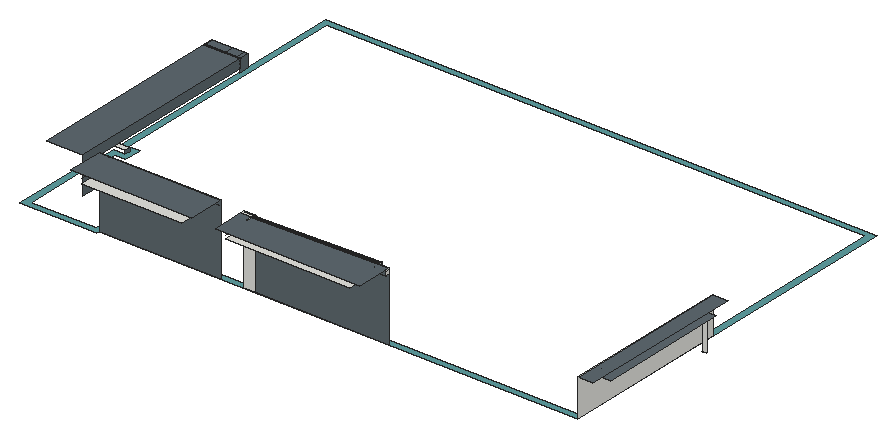
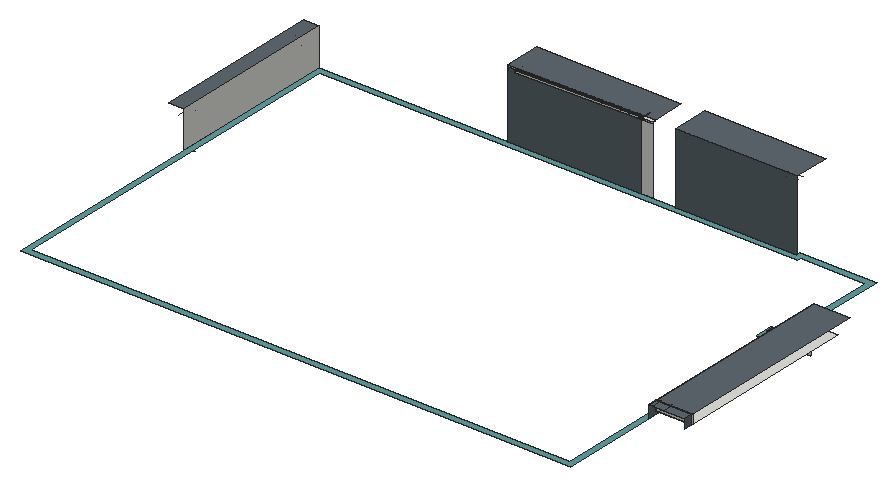
# SketchUp Ruby script. Lengths in inches.
U = 1.inch
M = Sketchup.active_model
def pt(a) = Geom::Point3d.new(a.map { |v| v * U })
def face(e, loops, mat)
  f = e.add_face(loops[0].map { |a| pt(a) })
  loops[1..].each { |l| e.add_face(l.map { |a| pt(a) }).erase! }
  f.material = f.back_material = mat if mat
  f
end
# faces: each face lists its corners as indices into pts; further lists are holes
def faces(e, pts, list, mat = nil) = list.each { |f| face(e, (f[0].is_a?(Array) ? f : [f]).map { |l| l.map { |i| pts[i] } }, mat) }
# xy, xz, yz: faces in a plane at the given z, y or x. An outline is a flat list of corners, or four numbers for a rectangle; further outlines are holes
def ring(l) = l.size == 4 ? [[l[0], l[1]], [l[2], l[1]], [l[2], l[3]], [l[0], l[3]]] : l.each_slice(2).to_a
def flat(e, list, mat, &to3) = list.each { |f| face(e, (f[0].is_a?(Array) ? f : [f]).map { |l| ring(l).map { |u, v| to3.(u, v) } }, mat) }
def xy(e, z, list, mat = nil) = flat(e, list, mat) { |x, y| [x, y, z] }
def xz(e, y, list, mat = nil) = flat(e, list, mat) { |x, z| [x, y, z] }
def yz(e, x, list, mat = nil) = flat(e, list, mat) { |y, z| [x, y, z] }
def lines(e, pts, list) = list.each { |a, b| e.add_line(pt(pts[a]), pt(pts[b])) }
# prism: a flat outline (further loops are holes) pulled along v
def prism(e, loops, v, mat = nil)
  f = face(e, loops, mat); d = Geom::Vector3d.new(v.map { |x| x * U })
  f.pushpull(f.normal.samedirection?(d) ? d.length : -d.length)
end
def box(e, o, s, mat = nil) = prism(e, [[o, [o[0] + s[0], o[1], o[2]], [o[0] + s[0], o[1] + s[1], o[2]], [o[0], o[1] + s[1], o[2]]]], [0, 0, s[2]], mat)
def at(x, y, z, deg = 0) = Geom::Transformation.translation(pt([x, y, z])) * Geom::Transformation.rotation(ORIGIN, Z_AXIS, deg.degrees)
def axes(o, x, y, z) = Geom::Transformation.new([*x, 0, *y, 0, *z, 0, *pt(o).to_a, 1])
def part(name) = M.definitions.add(name)
# library, detail: a bought-in or finely detailed component or shape, given as its bounding box
def library(name, o, s) = part(name).tap { |d| box(d.entities, o, s) }
def detail(e, o, s) = box(e.add_group.entities, o, s)
def put(e, d, t, mat = nil) = e.add_instance(d, t).tap { |i| i.material = mat if mat }
def group(e, t, mat = nil) = e.add_group.tap { |g| g.transformation = t; g.material = mat if mat }.entities
root = M.entities
M.materials.add("[0081_CadetBlue]").color = [95, 158, 160]
M.materials.add("[Formica Speckled Grey]").color = [94, 105, 111]
xy(root,684.183,[[[77.814,152.582,200.97,152.582,200.97,158.582,972.467,158.582,972.467,761.484,83.814,761.484,83.814,342.404,101.939,342.404,101.939,333.733,83.814,333.733,83.814,271.699,77.814,271.699],[86.814,161.582,86.814,262.699,92.814,262.699,92.814,324.733,110.939,324.733,110.939,351.404,92.814,351.404,92.814,752.484,963.467,752.484,963.467,167.582,191.97,167.582,191.97,161.582]]],"[0081_CadetBlue]")
xy(root,689.85,[[26.029,295.241,26.029,589.716,83.814,589.716,83.814,587.654,68.814,587.654,68.814,578.983,74.814,578.983,74.814,573.966,68.814,573.966,68.814,565.295,74.814,565.295,74.814,560.279,68.814,560.279,68.814,551.608,74.814,551.608,74.814,546.591,68.814,546.591,68.814,537.92,74.814,537.92,74.814,532.904,68.814,532.904,68.814,524.233,74.814,524.233,74.814,519.216,68.814,519.216,68.814,510.545,74.814,510.545,74.814,505.529,68.814,505.529,68.814,496.858,74.814,496.858,74.814,491.841,68.814,491.841,68.814,483.17,74.814,483.17,74.814,478.154,68.814,478.154,68.814,469.483,74.814,469.483,74.814,464.466,68.814,464.466,68.814,455.795,74.814,455.795,74.814,450.779,68.814,450.779,68.814,442.108,74.814,442.108,74.814,437.091,68.814,437.091,68.814,428.42,74.814,428.42,74.814,423.404,68.814,423.404,68.814,414.733,74.814,414.733,74.814,409.716,68.814,409.716,68.814,401.045,74.814,401.045,74.814,396.029,68.814,396.029,68.814,387.358,74.814,387.358,74.814,382.341,68.814,382.341,68.814,373.67,74.814,373.67,74.814,369.029,68.814,369.029,68.814,360.358,74.814,360.358,74.814,355.716,68.814,355.716,68.814,347.045,74.814,347.045,74.814,342.404,68.814,342.404,68.814,333.733,74.814,333.733,74.814,329.091,68.814,329.091,68.814,320.42,74.814,320.42,74.814,315.779,68.814,315.779,68.814,307.108,74.814,307.108,74.814,302.466,68.814,302.466,68.814,295.241],[68.814,295.241,74.814,302.466],[74.814,295.241,83.814,333.733],[68.814,307.108,74.814,315.779],[68.814,320.42,74.814,329.091],
  [68.814,333.733,74.814,342.404],[74.814,333.733,83.814,342.404],[83.814,333.733,101.939,342.404],[74.814,342.404,83.814,587.654],[68.814,347.045,74.814,355.716],
  [68.814,360.358,74.814,369.029],[68.814,373.67,74.814,382.341],[68.814,387.358,74.814,396.029],[68.814,401.045,74.814,409.716],[68.814,414.733,74.814,423.404],
  [68.814,428.42,74.814,437.091],[68.814,442.108,74.814,450.779],[68.814,455.795,74.814,464.466],[68.814,469.483,74.814,478.154],[68.814,483.17,74.814,491.841],
  [68.814,496.858,74.814,505.529],[68.814,510.545,74.814,519.216],[68.814,524.233,74.814,532.904],[68.814,537.92,74.814,546.591],[68.814,551.608,74.814,560.279],
  [68.814,565.295,74.814,573.966],[68.814,578.983,74.814,587.654]])
xy(root,704.683,[[26.029,271.699,83.814,587.654],[26.029,587.654,59.814,589.716],[59.814,587.654,77.814,589.716],[77.814,587.654,83.814,589.716],[26.029,589.716,59.814,604.3125],
  [59.814,589.716,77.814,604.3125],[77.814,589.716,83.814,604.3125]],"[Formica Speckled Grey]")
xy(root,732.183,[[974.717,194.926,980.717,205.629],[975.029,210.613,980.717,221.317],[975.029,226.301,980.717,237.004],[975.029,241.988,980.717,252.692],[975.029,257.676,980.717,268.379],
  [975.029,273.363,980.717,284.067],[975.029,289.051,980.717,299.754],[975.029,304.738,980.717,315.442],[975.029,320.426,980.717,331.129],[975.029,336.113,980.717,346.817],
  [975.029,351.801,981.029,362.504],[975.029,367.488,981.029,378.192],[975.029,383.176,981.029,393.879],[975.029,398.863,981.029,408.529]])
xy(root,732.183,[[980.717,194.926,980.717,205.629,975.029,205.629,975.029,210.613,980.717,210.613,980.717,221.317,975.029,221.317,975.029,226.301,980.717,226.301,980.717,237.004,975.029,237.004,975.029,241.988,980.717,241.988,980.717,252.692,975.029,252.692,975.029,257.676,980.717,257.676,980.717,268.379,975.029,268.379,975.029,273.363,980.717,273.363,980.717,284.067,975.029,284.067,975.029,289.051,980.717,289.051,980.717,299.754,975.029,299.754,975.029,304.738,980.717,304.738,980.717,315.442,975.029,315.442,975.029,320.426,980.717,320.426,980.717,331.129,975.029,331.129,975.029,336.113,980.717,336.113,980.717,346.817,975.029,346.817,975.029,351.801,981.029,351.801,981.029,362.504,975.029,362.504,975.029,367.488,981.029,367.488,981.029,378.192,975.029,378.192,975.029,383.176,981.029,383.176,981.029,393.879,975.029,393.879,975.029,398.863,981.029,398.863,981.029,408.529,996.467,408.529,996.467,194.926]],"[Formica Speckled Grey]")
xy(root,744.183,[[972.467,158.582,996.467,431.225]],"[Formica Speckled Grey]")
xy(root,784.183,[[217.792,100.797,217.792,140.582,223.26,140.582,223.26,137.582,231.22,137.582,231.22,140.582,235.635,140.582,235.635,137.582,243.595,137.582,243.595,140.582,248.01,140.582,248.01,137.582,255.97,137.582,255.97,140.582,260.385,140.582,260.385,137.582,268.345,137.582,268.345,140.582,272.76,140.582,272.76,137.582,280.72,137.582,280.72,140.582,285.135,140.582,285.135,137.582,293.095,137.582,293.095,140.582,297.51,140.582,297.51,137.582,305.47,137.582,305.47,140.582,309.885,140.582,309.885,137.582,317.845,137.582,317.845,140.582,322.26,140.582,322.26,137.582,330.22,137.582,330.22,140.582,334.635,140.582,334.635,137.582,342.595,137.582,342.595,140.582,347.01,140.582,347.01,137.582,354.97,137.582,354.97,140.582,359.385,140.582,359.385,137.582,367.345,137.582,367.345,140.582,371.76,140.582,371.76,137.582,379.72,137.582,379.72,100.797],[223.26,137.582,231.22,140.582],[235.635,137.582,243.595,140.582],[248.01,137.582,255.97,140.582],[260.385,137.582,268.345,140.582],
  [272.76,137.582,280.72,140.582],[285.135,137.582,293.095,140.582],[297.51,137.582,305.47,140.582],[309.885,137.582,317.845,140.582],[322.26,137.582,330.22,140.582],
  [334.635,137.582,342.595,140.582],[347.01,137.582,354.97,140.582],[359.385,137.582,367.345,140.582],[371.76,137.582,379.72,140.582],[217.792,140.582,217.792,143.582,379.72,143.582,379.72,140.582,305.47,140.582,305.47,140.894,297.51,140.894,297.51,140.582],
  [297.51,140.582,305.47,140.894],[217.792,143.582,379.72,146.582],[217.792,146.582,379.72,155.582]])
xy(root,786.183,[[450.855,100.797,450.855,152.582,451.124,143.586,451.214,140.587,460.874,140.877,460.784,143.875,651.119,149.574,651.119,143.76,645.312,143.586,645.388,141.034,651.119,141.206,651.119,100.797],[451.214,140.587,451.124,143.586,460.784,143.875,460.874,140.877],[645.388,141.034,645.312,143.586,651.119,143.76,651.119,141.206],[651.119,141.206,651.196,141.208,651.119,143.76],[651.196,141.208,655.048,141.323,654.971,143.875,651.119,143.76],
  [651.119,149.574,651.235,149.578,651.504,149.586,651.417,152.508,651.119,152.508]])
xy(root,792.183,[[451.124,143.586,651.235,149.578,650.967,158.523,450.856,152.531],[651.235,149.578,651.235,158.531,650.967,158.523],[651.235,149.578,651.235,158.531,651.237,158.531,651.504,149.586],[651.504,149.586,651.237,158.531,651.592,158.542,651.86,149.597],[668.057,152.508,668.057,158.519,667.692,152.53],
  [450.856,152.531,650.967,158.523,650.965,158.582,527.197,158.582,450.855,156.296,450.855,152.582],[450.855,152.582,450.744,156.293,450.855,156.296],[450.744,156.293,450.706,157.542,450.817,157.545,450.855,156.296],[450.855,156.296,450.817,157.545,450.855,157.547],[450.855,156.296,527.197,158.582,485.433,158.582,450.855,157.547],
  [450.706,157.542,450.682,158.354,450.793,158.358,450.817,157.545],[450.817,157.545,450.793,158.358,450.83,158.359,450.855,157.547],[450.855,157.547,450.83,158.359,450.855,158.359],[450.855,157.547,485.433,158.582,458.286,158.582,450.855,158.359],[450.855,158.359,458.286,158.582,450.855,158.582],
  [668.057,158.519,668.057,158.582,668.053,158.52],[650.967,158.523,650.965,158.582,651.233,158.582,651.235,158.531],[650.967,158.523,651.235,158.531,651.235,158.582,650.965,158.582],[651.235,158.531,651.233,158.582,651.235,158.582,651.237,158.531],[651.235,158.531,651.237,158.531,651.235,158.582],
  [651.237,158.531,651.235,158.582,651.591,158.582,651.592,158.542],[458.286,158.582,485.409,159.394,485.433,158.582],[485.433,158.582,485.409,159.394,527.136,160.644,527.16,159.831],[485.433,158.582,527.16,159.831,527.197,158.582],[527.197,158.582,527.16,159.831,650.817,163.534,650.855,162.285],
  [527.197,158.582,650.855,162.285,650.965,158.582],[650.965,158.582,650.855,162.285,651.122,162.293,651.233,158.582],[651.233,158.582,651.122,162.293,651.124,162.293,651.235,158.582],[651.235,158.582,651.124,162.293,651.479,162.303,651.591,158.582],[527.16,159.831,527.136,160.644,650.793,164.346,650.817,163.534],
  [650.855,162.285,650.817,163.534,651.085,163.542,651.122,162.293],[651.122,162.293,651.085,163.542,651.086,163.542,651.124,162.293],[651.124,162.293,651.086,163.542,651.442,163.553,651.479,162.303],[650.817,163.534,650.793,164.346,651.061,164.354,651.085,163.542],[651.085,163.542,651.061,164.354,651.062,164.354,651.086,163.542],
  [651.086,163.542,651.062,164.354,651.417,164.365,651.442,163.553]])
xy(root,795.183,[[450.856,152.531,651.237,158.531,651.235,158.582,651.124,162.293,450.855,156.296,450.855,152.582],[434.033,152.582,450.855,152.582,450.744,156.293,450.706,157.542,450.682,158.354,450.793,158.358,450.83,158.359,450.855,158.359,450.855,158.582,434.033,158.582],[450.855,152.582,450.855,156.296,450.744,156.293],[450.744,156.293,450.855,156.296,450.817,157.545,450.706,157.542],[450.855,156.296,450.855,157.547,450.817,157.545],
  [450.855,156.296,651.124,162.293,651.086,163.542,450.855,157.547],[450.706,157.542,450.817,157.545,450.793,158.358,450.682,158.354],[450.817,157.545,450.855,157.547,450.83,158.359,450.793,158.358],[450.855,157.547,450.855,158.359,450.83,158.359],[450.855,157.547,651.086,163.542,651.062,164.354,450.855,158.359],
  [651.237,158.531,651.592,158.542,651.591,158.582,651.235,158.582],[651.235,158.582,651.591,158.582,651.479,162.303,651.124,162.293],[651.124,162.293,651.479,162.303,651.442,163.553,651.086,163.542],[651.086,163.542,651.442,163.553,651.417,164.365,651.062,164.354]])
xy(root,795.183,[[434.033,100.797,668.057,100.797,668.057,152.508,667.692,152.53,668.057,158.519,668.053,158.52,668.057,158.582,651.591,158.582,651.592,158.542,651.237,158.531,450.856,152.531,450.855,152.582,434.033,152.582]],"[Formica Speckled Grey]")
xy(root,798.183,[[200.97,100.797,396.542,158.582]],"[Formica Speckled Grey]")
xz(root,155.582,[[217.792,784.183,379.72,792.183]])
xz(root,158.582,[[434.033,684.183,450.855,792.183],[434.033,792.183,450.855,795.183],[651.235,792.183,668.057,795.183]])
xz(root,158.582,[[200.97,684.183,396.542,798.183],[450.855,684.183,668.057,792.183]],"[Formica Speckled Grey]")
xz(root,295.241,[[68.814,644.683,74.814,689.85],[74.814,644.683,83.814,689.85]])
xz(root,408.529,[[975.029,672.183,981.029,732.183]])
xz(root,589.716,[[26.029,689.85,77.814,704.683],[77.814,689.85,83.814,704.683]])
yz(root,26.029,[[587.654,689.85,589.716,704.683]])
yz(root,26.029,[[589.716,689.85,604.3125,704.683]],"[Formica Speckled Grey]")
yz(root,83.814,[[587.654,689.85,589.716,704.683]])
yz(root,83.814,[[271.699,644.683,295.241,684.183],[271.699,684.183,295.241,684.183,295.241,689.85,587.654,689.85,587.654,704.683,271.699,704.683],[587.654,684.183,604.3125,684.183,604.3125,704.683,589.716,704.683,589.716,689.85,587.654,689.85]],"[Formica Speckled Grey]")
yz(root,101.939,[[333.733,684.183,342.404,689.85]],"[Formica Speckled Grey]")
yz(root,217.792,[[146.582,784.183,155.582,792.183]])
yz(root,450.855,[[152.582,792.183,158.582,795.183]])
yz(root,972.467,[[158.582,684.183,431.225,744.183]])
p = [[450.856,152.531,792.183],[450.855,152.582,792.183],[450.855,152.582,786.183],[451.124,143.586,786.183],[451.124,143.586,792.183],[651.235,149.578,792.183],
  [460.784,143.875,786.183],[651.119,149.574,786.183],[651.235,149.578,786.183],[651.504,149.586,792.183],[651.504,149.586,786.183],[667.692,152.53,792.183],
  [668.057,152.508,792.183],[668.057,152.508,786.183],[667.692,152.53,786.183],[668.057,158.519,792.183],[668.057,158.519,786.183],[668.053,158.52,792.183],
  [668.053,158.52,786.183],[668.057,158.582,792.183],[668.057,158.582,786.183],[451.124,143.586,795.183],[450.856,152.531,795.183],[450.855,152.582,795.183],
  [651.237,158.531,795.183],[650.967,158.523,792.183],[651.235,158.531,792.183],[651.237,158.531,792.183],[651.592,158.542,792.183],[651.592,158.542,795.183],
  [667.692,152.53,795.183],[668.057,152.508,795.183],[668.057,158.519,795.183],[450.744,156.293,792.183],[450.744,156.293,795.183],[651.124,162.293,795.183],
  [450.855,156.296,795.183],[450.855,156.296,792.183],[527.197,158.582,792.183],[650.855,162.285,792.183],[651.122,162.293,792.183],[651.124,162.293,792.183],
  [651.479,162.303,792.183],[651.479,162.303,795.183],[450.706,157.542,795.183],[450.706,157.542,792.183],[450.682,158.354,795.183],[450.682,158.354,792.183],
  [651.086,163.542,795.183],[450.855,157.547,795.183],[450.817,157.545,795.183],[450.817,157.545,792.183],[450.855,157.547,792.183],[485.433,158.582,792.183],
  [527.16,159.831,792.183],[650.817,163.534,792.183],[651.085,163.542,792.183],[651.086,163.542,792.183],[651.442,163.553,792.183],[651.442,163.553,795.183],
  [450.855,158.359,795.183],[651.062,164.354,795.183],[651.417,164.365,795.183],[651.417,164.365,792.183],[651.062,164.354,792.183],[651.061,164.354,792.183],
  [650.793,164.346,792.183],[527.136,160.644,792.183],[485.409,159.394,792.183],[458.286,158.582,792.183],[450.855,158.359,792.183],[450.83,158.359,792.183],
  [450.793,158.358,792.183],[450.793,158.358,795.183],[450.83,158.359,795.183],[651.591,158.582,792.183],[651.591,158.582,795.183],[668.053,158.52,795.183],
  [668.057,158.582,795.183],[217.792,146.582,792.183],[217.792,100.797,792.183],[217.792,155.582,792.183],[217.792,155.582,798.183],[379.72,155.582,792.183],
  [396.542,155.582,792.183],[200.97,146.582,792.183],[200.97,155.582,792.183],[217.792,158.582,792.183],[379.72,158.582,792.183],[450.855,100.797,792.183],
  [651.235,158.582,786.183],[651.417,152.508,786.183],[651.235,149.578,795.183],[434.033,152.582,792.183],[651.86,149.597,792.183],[651.86,149.597,795.183],
  [77.814,589.716,689.85],[77.814,604.3125,689.85],[981.467,194.926,732.183],[981.467,194.926,744.183],[981.467,408.529,732.183],[981.467,431.225,732.183],
  [972.467,408.529,672.183],[975.029,408.529,672.183],[975.029,408.529,732.183],[972.467,408.529,732.183],[974.717,194.926,732.183],[972.467,194.926,732.183]]
faces(root,p,[[0,1,2,3,4],[5,4,3,6,7,8],[9,5,8,10],[11,12,13,14],[15,11,14,16],[17,15,16,18],[19,17,18,20],[21,4,0,22],
  [1,0,22,23],[24,22,0,25,26,27,28,29],[12,11,30,31],[11,15,32,30],[33,1,23,34],[35,36,34,33,37,38,39,40,41,42,43],[33,34,44,45],[45,44,46,47],
  [48,49,50,44,45,51,52,53,54,55,56,57,58,59],[60,61,62,63,64,65,66,67,68,69,70,71,72,47,46,73,74],[29,28,75,42,43,76],[15,17,77,32],[17,19,78,77],[43,42,58,59],[59,58,63,62]])
lines(root,p,[[79,80],[81,82],[83,84],[79,85],[81,86],[81,87],[83,88],[1,89],[90,91],[5,92],[1,93],[13,91],
  [94,95],[96,97],[98,99],[100,101],[102,103],[104,105],[106,107]])
